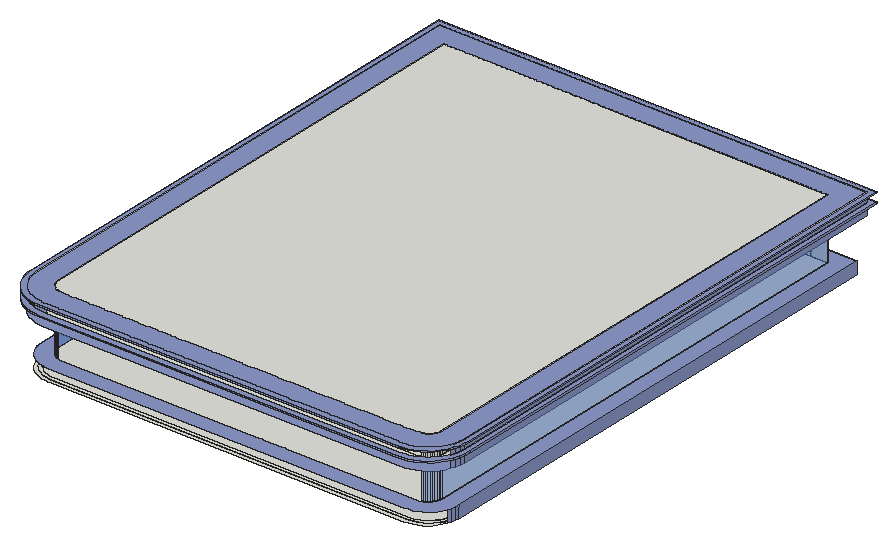
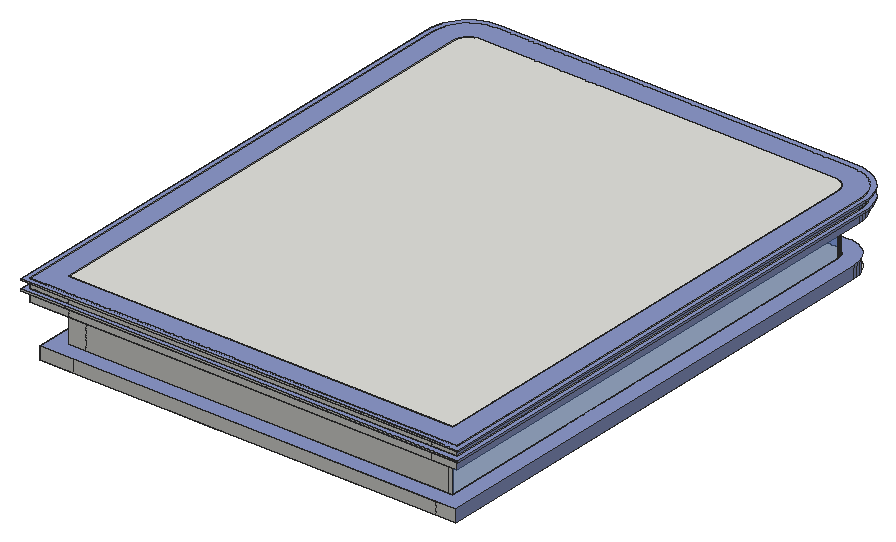
# SketchUp Ruby script. Lengths in inches.
U = 1.inch
M = Sketchup.active_model
def pt(a) = Geom::Point3d.new(a.map { |v| v * U })
def face(e, loops, mat)
  f = e.add_face(loops[0].map { |a| pt(a) })
  loops[1..].each { |l| e.add_face(l.map { |a| pt(a) }).erase! }
  f.material = f.back_material = mat if mat
  f
end
# faces: each face lists its corners as indices into pts; further lists are holes
def faces(e, pts, list, mat = nil) = list.each { |f| face(e, (f[0].is_a?(Array) ? f : [f]).map { |l| l.map { |i| pts[i] } }, mat) }
# xy, xz, yz: faces in a plane at the given z, y or x. An outline is a flat list of corners, or four numbers for a rectangle; further outlines are holes
def ring(l) = l.size == 4 ? [[l[0], l[1]], [l[2], l[1]], [l[2], l[3]], [l[0], l[3]]] : l.each_slice(2).to_a
def flat(e, list, mat, &to3) = list.each { |f| face(e, (f[0].is_a?(Array) ? f : [f]).map { |l| ring(l).map { |u, v| to3.(u, v) } }, mat) }
def xy(e, z, list, mat = nil) = flat(e, list, mat) { |x, y| [x, y, z] }
def xz(e, y, list, mat = nil) = flat(e, list, mat) { |x, z| [x, y, z] }
def yz(e, x, list, mat = nil) = flat(e, list, mat) { |y, z| [x, y, z] }
def lines(e, pts, list) = list.each { |a, b| e.add_line(pt(pts[a]), pt(pts[b])) }
# prism: a flat outline (further loops are holes) pulled along v
def prism(e, loops, v, mat = nil)
  f = face(e, loops, mat); d = Geom::Vector3d.new(v.map { |x| x * U })
  f.pushpull(f.normal.samedirection?(d) ? d.length : -d.length)
end
def box(e, o, s, mat = nil) = prism(e, [[o, [o[0] + s[0], o[1], o[2]], [o[0] + s[0], o[1] + s[1], o[2]], [o[0], o[1] + s[1], o[2]]]], [0, 0, s[2]], mat)
def at(x, y, z, deg = 0) = Geom::Transformation.translation(pt([x, y, z])) * Geom::Transformation.rotation(ORIGIN, Z_AXIS, deg.degrees)
def axes(o, x, y, z) = Geom::Transformation.new([*x, 0, *y, 0, *z, 0, *pt(o).to_a, 1])
def part(name) = M.definitions.add(name)
# library, detail: a bought-in or finely detailed component or shape, given as its bounding box
def library(name, o, s) = part(name).tap { |d| box(d.entities, o, s) }
def detail(e, o, s) = box(e.add_group.entities, o, s)
def put(e, d, t, mat = nil) = e.add_instance(d, t).tap { |i| i.material = mat if mat }
def group(e, t, mat = nil) = e.add_group.tap { |g| g.transformation = t; g.material = mat if mat }.entities
root = M.entities
M.materials.add("0326 AP 7207 CLASSIC PURPLE").color = [140, 152, 201]
M.materials.add("[Translucent Glass Blue]").color = [100, 149, 237]
M.materials["[Translucent Glass Blue]"].alpha = 0.5
xy(root,372,[[[167.6875,42.4375,166.41,42.52,163.74,42.7,159.87,43.47,157.41,44.3,156.125,44.74,152.58,46.49,149.29,48.68,146.32,51.29,143.71,54.26,141.52,57.55,139.77,61.09,138.5,64.84,137.73,68.71,137.47,72.66,137.47,233.75,247.2,233.75,247.2,141.25,257.02,141.25,257.02,224.35,364.41,224.35,364.41,86.25,517.41,86.25,517.41,566.25,550.66,566.25,550.66,72.66,550.4,68.71,549.63,64.84,548.36,61.09,546.61,57.55,544.41,54.26,541.81,51.29,538.83,48.68,535.55,46.49,532,44.74,528.26,43.47,524.38,42.7,520.4375,42.4375],[167.8,45.71,520.4375,45.71,523.96,45.9375,527.41,46.625,530.75,47.76,533.91,49.32,536.84,51.28,539.49,53.6,541.82,56.25,543.78,59.18,545.34,62.34,546.47,65.68,547.16,69.14,547.39,72.66,547.39,176.17,544.33,176.17,544.33,72.66,544.12,69.54,543.51,66.47,542.51,63.51,541.125,60.71,539.39,58.11,537.33,55.76,534.98,53.7,532.38,51.97,529.58,50.59,526.62,49.58,523.56,48.97,520.4375,48.77,167.9,48.77,166.82,48.84,164.57,48.98,161.51,49.59,159.44,50.3,158.55,50.6,155.75,51.98,153.15,53.71,150.81,55.77,148.75,58.12,147.01,60.72,145.63,63.52,144.625,66.48,144.02,69.54,143.8,72.86,143.8,227.42,140.74,230.48,140.74,72.76,140.98,69.14,141.66,65.68,142.8,62.35,144.36,59.1875,146.3125,56.26,148.64,53.61,151.29,51.28,154.22,49.32,157.38,47.77,158.46,47.4,160.72,46.63,164.17,45.95,166.62,45.78]],[364.41,86.25,373.41,566.25],[373.41,86.25,508.41,95.25],[508.41,86.25,517.41,95.25],[373.41,95.25,508.41,557.25],
  [508.41,95.25,517.41,566.25],[247.2,141.25,257.02,566.25],[257.02,224.35,364.41,238.8],[137.47,233.75,157.41,566.25],[157.41,233.75,166.41,566.25],
  [166.41,233.75,247.2,252.68],[257.02,238.8,364.41,566.25],[166.41,252.68,247.2,566.25],[373.41,557.25,508.41,566.25]])
xy(root,372.8125,[[167.8,45.71,166.62,45.78,164.17,45.95,160.72,46.63,158.46,47.4,157.38,47.77,154.22,49.32,151.29,51.28,148.64,53.61,146.3125,56.26,144.36,59.1875,142.8,62.35,141.66,65.68,140.98,69.14,140.74,72.76,140.74,230.48,143.8,227.42,143.8,72.86,144.02,69.54,144.625,66.48,145.63,63.52,147.01,60.72,148.75,58.12,150.81,55.77,153.15,53.71,155.75,51.98,158.55,50.6,159.44,50.3,161.51,49.59,164.57,48.98,166.82,48.84,167.9,48.77,520.4375,48.77,523.56,48.97,526.62,49.58,529.58,50.59,532.38,51.97,534.98,53.7,537.33,55.76,539.39,58.11,541.125,60.71,542.51,63.51,543.51,66.47,544.12,69.54,544.33,72.66,544.33,176.17,547.39,176.17,547.39,72.66,547.16,69.14,546.47,65.68,545.34,62.34,543.78,59.18,541.82,56.25,539.49,53.6,536.84,51.28,533.91,49.32,530.75,47.76,527.41,46.625,523.96,45.9375,520.4375,45.71]])
xy(root,384,[[168.22,58.64,165.86,58.8,164.07,59.15,162.62,59.65,162.34,59.74,160.7,60.55,159.18,61.57,157.8,62.77,156.6,64.15,155.58,65.67,154.77,67.31,154.1875,69.04,153.83,70.83,153.68,73.1875,153.68,550.04,534.45,550.04,534.45,72.66,534.33,70.83,533.97,69.03,533.38,67.29,532.57,65.65,531.56,64.125,530.35,62.75,528.97,61.54,527.44,60.52,525.8,59.71,524.06,59.12,522.27,58.76,520.4375,58.64]])
xy(root,384,[[[167.6875,42.4375,520.4375,42.4375,524.38,42.7,528.26,43.47,532,44.74,535.55,46.49,538.83,48.68,541.81,51.29,544.41,54.26,546.61,57.55,548.36,61.09,549.63,64.84,550.4,68.71,550.66,72.66,550.66,566.25,137.47,566.25,137.47,72.66,137.73,68.71,138.5,64.84,139.77,61.09,141.52,57.55,143.71,54.26,146.32,51.29,149.29,48.68,152.58,46.49,156.125,44.74,157.41,44.3,159.87,43.47,163.74,42.7],[168.22,58.64,165.86,58.8,164.07,59.15,162.62,59.65,162.34,59.74,160.7,60.55,159.18,61.57,157.8,62.77,156.6,64.15,155.58,65.67,154.77,67.31,154.1875,69.04,153.83,70.83,153.68,73.1875,153.68,550.04,534.45,550.04,534.45,72.66,534.33,70.83,533.97,69.03,533.38,67.29,532.57,65.65,531.56,64.125,530.35,62.75,528.97,61.54,527.44,60.52,525.8,59.71,524.06,59.12,522.27,58.76,520.4375,58.64]]],"0326 AP 7207 CLASSIC PURPLE")
xy(root,420.75,[[[168.01,52.13,165.01,52.33,162.38,52.85,160.52,53.48,159.84,53.72,157.4375,54.9,155.21,56.39,153.19,58.16,151.42,60.18,149.93,62.41,148.75,64.8125,147.89,67.35,147.36,69.98,147.17,72.97,147.17,556.55,540.96,556.55,540.96,72.66,540.78,69.98,540.26,67.34,539.4,64.8,538.21,62.4,536.72,60.16,534.95,58.15,532.93,56.375,530.7,54.88,528.29,53.7,525.75,52.83,523.12,52.31,520.4375,52.13],[168.22,58.64,520.4375,58.64,522.27,58.76,524.06,59.12,525.8,59.71,527.44,60.52,528.97,61.54,530.35,62.75,531.56,64.125,532.57,65.65,533.38,67.29,533.97,69.03,534.33,70.83,534.45,72.66,534.45,550.04,153.68,550.04,153.68,73.1875,153.83,70.83,154.1875,69.04,154.77,67.31,155.58,65.67,156.6,64.15,157.8,62.77,159.18,61.57,160.7,60.55,162.34,59.74,162.62,59.65,164.07,59.15,165.86,58.8]]],"0326 AP 7207 CLASSIC PURPLE")
xy(root,423.4375,[[[168.01,52.13,520.4375,52.13,523.12,52.31,525.75,52.83,528.29,53.7,530.7,54.88,532.93,56.375,534.95,58.15,536.72,60.16,538.21,62.4,539.4,64.8,540.26,67.34,540.78,69.98,540.96,72.66,540.96,556.55,147.17,556.55,147.17,72.97,147.36,69.98,147.89,67.35,148.75,64.8125,149.93,62.41,151.42,60.18,153.19,58.16,155.21,56.39,157.4375,54.9,159.84,53.72,160.52,53.48,162.38,52.85,165.01,52.33],[168.22,58.64,165.86,58.8,164.07,59.15,162.62,59.65,162.34,59.74,160.7,60.55,159.18,61.57,157.8,62.77,156.6,64.15,155.58,65.67,154.77,67.31,154.1875,69.04,153.83,70.83,153.68,73.1875,153.68,550.04,534.45,550.04,534.45,72.66,534.33,70.83,533.97,69.03,533.38,67.29,532.57,65.65,531.56,64.125,530.35,62.75,528.97,61.54,527.44,60.52,525.8,59.71,524.06,59.12,522.27,58.76,520.4375,58.64]]])
xy(root,423.4375,[[[167.51,37.02,163.03,37.3125,158.46,38.22,155.67,39.17,154.05,39.72,149.86,41.78,145.99,44.375,142.48,47.45,139.41,50.95,136.82,54.83,134.75,59.01,133.25,63.43,132.34,68,132.05,72.48,132.05,571.67,556.08,571.67,556.08,72.66,555.77,68,554.86,63.43,553.36,59.02,551.3,54.84,548.71,50.96,545.64,47.46,542.13,44.38,538.26,41.79,534.08,39.73,529.66,38.23,525.09,37.32,520.4375,37.02],[168.01,52.13,520.4375,52.13,523.12,52.31,525.75,52.83,528.29,53.7,530.7,54.88,532.93,56.375,534.95,58.15,536.72,60.16,538.21,62.4,539.4,64.8,540.26,67.34,540.78,69.98,540.96,72.66,540.96,556.55,147.17,556.55,147.17,72.97,147.36,69.98,147.89,67.35,148.75,64.8125,149.93,62.41,151.42,60.18,153.19,58.16,155.21,56.39,157.4375,54.9,159.84,53.72,160.52,53.48,162.38,52.85,165.01,52.33]]],"0326 AP 7207 CLASSIC PURPLE")
xy(root,433.9375,[[[167.34,31.9,162.36,32.22,157.13,33.26,154.02,34.32,152.08,34.98,147.3,37.34,142.86,40.3,138.85,43.82,135.33,47.83,132.37,52.26,130.01,57.05,128.29,62.1,127.25,67.33,126.93,72.3125,126.93,576.79,561.2,576.79,561.2,72.66,560.85,67.34,559.81,62.11,558.1,57.06,555.74,52.28,552.78,47.84,549.26,43.83,545.25,40.32,540.82,37.36,536.04,35,530.99,33.28,525.76,32.24,520.4375,31.9],[167.51,37.02,520.4375,37.02,525.09,37.32,529.66,38.23,534.08,39.73,538.26,41.79,542.13,44.38,545.64,47.46,548.71,50.96,551.3,54.84,553.36,59.02,554.86,63.43,555.77,68,556.08,72.66,556.08,571.67,132.05,571.67,132.05,72.48,132.34,68,133.25,63.43,134.75,59.01,136.82,54.83,139.41,50.95,142.48,47.45,145.99,44.375,149.86,41.78,154.05,39.72,155.67,39.17,158.46,38.22,163.03,37.3125]]],"0326 AP 7207 CLASSIC PURPLE")
xy(root,435.625,[[[167.34,31.9,520.4375,31.9,525.76,32.24,530.99,33.28,536.04,35,540.82,37.36,545.25,40.32,549.26,43.83,552.78,47.84,555.74,52.28,558.1,57.06,559.81,62.11,560.85,67.34,561.2,72.66,561.2,576.79,126.93,576.79,126.93,72.3125,127.25,67.33,128.29,62.1,130.01,57.05,132.37,52.26,135.33,47.83,138.85,43.82,142.86,40.3,147.3,37.34,152.08,34.98,154.02,34.32,157.13,33.26,162.36,32.22],[167.51,37.02,163.03,37.3125,158.46,38.22,155.67,39.17,154.05,39.72,149.86,41.78,145.99,44.375,142.48,47.45,139.41,50.95,136.82,54.83,134.75,59.01,133.25,63.43,132.34,68,132.05,72.48,132.05,571.67,556.08,571.67,556.08,72.66,555.77,68,554.86,63.43,553.36,59.02,551.3,54.84,548.71,50.96,545.64,47.46,542.13,44.38,538.26,41.79,534.08,39.73,529.66,38.23,525.09,37.32,520.4375,37.02]]],"0326 AP 7207 CLASSIC PURPLE")
xy(root,443.3125,[[[167.34,31.9,162.36,32.22,157.13,33.26,154.02,34.32,152.08,34.98,147.3,37.34,142.86,40.3,138.85,43.82,135.33,47.83,132.37,52.26,130.01,57.05,128.29,62.1,127.25,67.33,126.93,72.3125,126.93,576.79,561.2,576.79,561.2,72.66,560.85,67.34,559.81,62.11,558.1,57.06,555.74,52.28,552.78,47.84,549.26,43.83,545.25,40.32,540.82,37.36,536.04,35,530.99,33.28,525.76,32.24,520.4375,31.9],[167.51,37.02,520.4375,37.02,525.09,37.32,529.66,38.23,534.08,39.73,538.26,41.79,542.13,44.38,545.64,47.46,548.71,50.96,551.3,54.84,553.36,59.02,554.86,63.43,555.77,68,556.08,72.66,556.08,571.67,132.05,571.67,132.05,72.48,132.34,68,133.25,63.43,134.75,59.01,136.82,54.83,139.41,50.95,142.48,47.45,145.99,44.375,149.86,41.78,154.05,39.72,155.67,39.17,158.46,38.22,163.03,37.3125]]],"0326 AP 7207 CLASSIC PURPLE")
xy(root,444.625,[[168.22,58.64,520.4375,58.64,522.27,58.76,524.06,59.12,525.8,59.71,527.44,60.52,528.97,61.54,530.35,62.75,531.56,64.125,532.57,65.65,533.38,67.29,533.97,69.03,534.33,70.83,534.45,72.66,534.45,550.04,153.68,550.04,153.68,73.1875,153.83,70.83,154.1875,69.04,154.77,67.31,155.58,65.67,156.6,64.15,157.8,62.77,159.18,61.57,160.7,60.55,162.34,59.74,162.62,59.65,164.07,59.15,165.86,58.8]])
xy(root,444.625,[[[167.34,31.9,520.4375,31.9,525.76,32.24,530.99,33.28,536.04,35,540.82,37.36,545.25,40.32,549.26,43.83,552.78,47.84,555.74,52.28,558.1,57.06,559.81,62.11,560.85,67.34,561.2,72.66,561.2,576.79,126.93,576.79,126.93,72.3125,127.25,67.33,128.29,62.1,130.01,57.05,132.37,52.26,135.33,47.83,138.85,43.82,142.86,40.3,147.3,37.34,152.08,34.98,154.02,34.32,157.13,33.26,162.36,32.22],[167.51,37.02,163.03,37.3125,158.46,38.22,155.67,39.17,154.05,39.72,149.86,41.78,145.99,44.375,142.48,47.45,139.41,50.95,136.82,54.83,134.75,59.01,133.25,63.43,132.34,68,132.05,72.48,132.05,571.67,556.08,571.67,556.08,72.66,555.77,68,554.86,63.43,553.36,59.02,551.3,54.84,548.71,50.96,545.64,47.46,542.13,44.38,538.26,41.79,534.08,39.73,529.66,38.23,525.09,37.32,520.4375,37.02]],[[167.51,37.02,520.4375,37.02,525.09,37.32,529.66,38.23,534.08,39.73,538.26,41.79,542.13,44.38,545.64,47.46,548.71,50.96,551.3,54.84,553.36,59.02,554.86,63.43,555.77,68,556.08,72.66,556.08,571.67,132.05,571.67,132.05,72.48,132.34,68,133.25,63.43,134.75,59.01,136.82,54.83,139.41,50.95,142.48,47.45,145.99,44.375,149.86,41.78,154.05,39.72,155.67,39.17,158.46,38.22,163.03,37.3125],[168.22,58.64,165.86,58.8,164.07,59.15,162.62,59.65,162.34,59.74,160.7,60.55,159.18,61.57,157.8,62.77,156.6,64.15,155.58,65.67,154.77,67.31,154.1875,69.04,153.83,70.83,153.68,73.1875,153.68,550.04,534.45,550.04,534.45,72.66,534.33,70.83,533.97,69.03,533.38,67.29,532.57,65.65,531.56,64.125,530.35,62.75,528.97,61.54,527.44,60.52,525.8,59.71,524.06,59.12,522.27,58.76,520.4375,58.64]]],"0326 AP 7207 CLASSIC PURPLE")
xz(root,176.17,[[544.33,372,547.39,372.8125]])
xz(root,550.04,[[153.68,384,157.41,420.75],[157.41,384,517.41,420.75],[517.41,384,534.45,420.75],[153.68,420.75,157.41,423.4375],[157.41,420.75,517.41,423.4375],
  [517.41,420.75,534.45,423.4375],[153.68,423.4375,157.41,444.625],[157.41,423.4375,517.41,444.625],[517.41,423.4375,534.45,444.625]])
xz(root,556.55,[[147.17,420.75,157.41,423.4375],[157.41,420.75,517.41,423.4375],[517.41,420.75,540.96,423.4375]])
xz(root,566.25,[[137.47,372,157.41,384],[157.41,372,517.41,384],[517.41,372,550.66,384]])
xz(root,571.67,[[132.05,423.4375,157.41,433.9375],[157.41,423.4375,517.41,433.9375],[517.41,423.4375,556.08,433.9375],[132.05,433.9375,157.41,435.625],[157.41,433.9375,517.41,435.625],
  [517.41,433.9375,556.08,435.625],[132.05,435.625,157.41,443.3125],[157.41,435.625,517.41,443.3125],[517.41,435.625,556.08,443.3125],[132.05,443.3125,157.41,444.625],
  [157.41,443.3125,517.41,444.625],[517.41,443.3125,556.08,444.625]])
xz(root,576.79,[[126.93,433.9375,157.41,435.625],[157.41,433.9375,517.41,435.625],[517.41,433.9375,561.2,435.625],[126.93,443.3125,157.41,444.625],[157.41,443.3125,517.41,444.625],
  [517.41,443.3125,561.2,444.625]])
yz(root,126.93,[[72.3125,433.9375,576.79,435.625],[72.3125,443.3125,576.79,444.625]],"0326 AP 7207 CLASSIC PURPLE")
yz(root,132.05,[[72.48,433.9375,571.67,435.625],[72.48,443.3125,571.67,444.625]])
yz(root,132.05,[[72.48,423.4375,571.67,433.9375],[72.48,435.625,571.67,443.3125]],"0326 AP 7207 CLASSIC PURPLE")
yz(root,137.47,[[72.66,372,566.25,384]],"0326 AP 7207 CLASSIC PURPLE")
yz(root,140.74,[[72.76,372,230.48,372.8125]])
yz(root,143.8,[[72.86,372,227.42,372.8125]])
yz(root,147.17,[[72.97,420.75,556.55,423.4375]],"0326 AP 7207 CLASSIC PURPLE")
yz(root,153.68,[[73.1875,420.75,550.04,423.4375],[73.1875,423.4375,550.04,444.625]])
yz(root,153.68,[[73.1875,384,550.04,420.75]],"[Translucent Glass Blue]")
yz(root,534.45,[[72.66,420.75,550.04,423.4375],[72.66,423.4375,550.04,444.625]])
yz(root,534.45,[[72.66,384,550.04,420.75]],"[Translucent Glass Blue]")
yz(root,540.96,[[72.66,420.75,556.55,423.4375]],"0326 AP 7207 CLASSIC PURPLE")
yz(root,544.33,[[72.66,372,176.17,372.8125]])
yz(root,547.39,[[72.66,372,176.17,372.8125]])
yz(root,550.66,[[72.66,372,566.25,384]],"0326 AP 7207 CLASSIC PURPLE")
yz(root,556.08,[[72.66,433.9375,571.67,435.625],[72.66,443.3125,571.67,444.625]])
yz(root,556.08,[[72.66,423.4375,571.67,433.9375],[72.66,435.625,571.67,443.3125]],"0326 AP 7207 CLASSIC PURPLE")
yz(root,561.2,[[72.66,433.9375,576.79,435.625],[72.66,443.3125,576.79,444.625]],"0326 AP 7207 CLASSIC PURPLE")
p = [[147.01,60.72,372],[148.75,58.12,372],[148.75,58.12,372.8125],[147.01,60.72,372.8125],[539.39,58.11,372],[541.125,60.71,372],
  [541.125,60.71,372.8125],[539.39,58.11,372.8125],[144.36,59.1875,372],[142.8,62.35,372],[142.8,62.35,372.8125],[144.36,59.1875,372.8125],
  [545.34,62.34,372],[543.78,59.18,372],[543.78,59.18,372.8125],[545.34,62.34,372.8125],[145.63,63.52,372],[145.63,63.52,372.8125],
  [542.51,63.51,372],[542.51,63.51,372.8125],[139.77,61.09,384],[138.5,64.84,384],[138.5,64.84,372],[139.77,61.09,372],
  [549.63,64.84,384],[548.36,61.09,384],[548.36,61.09,372],[549.63,64.84,372],[141.66,65.68,372],[141.66,65.68,372.8125],
  [546.47,65.68,372],[546.47,65.68,372.8125],[144.625,66.48,372],[144.625,66.48,372.8125],[543.51,66.47,372],[543.51,66.47,372.8125],
  [137.73,68.71,384],[137.73,68.71,372],[550.4,68.71,384],[550.4,68.71,372],[140.98,69.14,372],[140.98,69.14,372.8125],
  [547.16,69.14,372],[547.16,69.14,372.8125],[144.02,69.54,372],[144.02,69.54,372.8125],[544.12,69.54,372],[544.12,69.54,372.8125],
  [137.47,72.66,384],[137.47,72.66,372],[550.66,72.66,384],[550.66,72.66,372],[140.74,72.76,372],[140.74,72.76,372.8125],
  [547.39,72.66,372],[547.39,72.66,372.8125],[143.8,72.86,372],[143.8,72.86,372.8125],[544.33,72.66,372],[544.33,72.66,372.8125],
  [140.74,230.48,372],[143.8,227.42,372],[143.8,227.42,372.8125],[140.74,230.48,372.8125],[524.06,59.12,384],[525.8,59.71,384],
  [525.8,59.71,420.75],[524.06,59.12,420.75],[162.62,59.65,384],[164.07,59.15,384],[164.07,59.15,420.75],[162.62,59.65,420.75],
  [162.34,59.74,384],[162.34,59.74,420.75],[160.7,60.55,384],[160.7,60.55,420.75],[527.44,60.52,384],[527.44,60.52,420.75],
  [528.97,61.54,384],[528.97,61.54,420.75],[159.18,61.57,384],[159.18,61.57,420.75],[530.35,62.75,384],[530.35,62.75,420.75],
  [157.8,62.77,384],[157.8,62.77,420.75],[531.56,64.125,384],[531.56,64.125,420.75],[156.6,64.15,384],[156.6,64.15,420.75],
  [155.58,65.67,384],[155.58,65.67,420.75],[532.57,65.65,384],[532.57,65.65,420.75],[533.38,67.29,384],[533.38,67.29,420.75],
  [154.77,67.31,384],[154.77,67.31,420.75],[154.1875,69.04,384],[154.1875,69.04,420.75],[533.97,69.03,384],[533.97,69.03,420.75],
  [153.83,70.83,384],[153.83,70.83,420.75],[534.33,70.83,384],[534.33,70.83,420.75],[153.68,73.1875,384],[153.68,73.1875,420.75],
  [534.45,72.66,384],[534.45,72.66,420.75],[525.8,59.71,423.4375],[524.06,59.12,423.4375],[164.07,59.15,423.4375],[162.62,59.65,423.4375],
  [162.34,59.74,423.4375],[160.7,60.55,423.4375],[527.44,60.52,423.4375],[151.42,60.18,423.4375],[149.93,62.41,423.4375],[149.93,62.41,420.75],
  [151.42,60.18,420.75],[538.21,62.4,423.4375],[536.72,60.16,423.4375],[536.72,60.16,420.75],[538.21,62.4,420.75],[528.97,61.54,423.4375],
  [159.18,61.57,423.4375],[530.35,62.75,423.4375],[157.8,62.77,423.4375],[148.75,64.8125,423.4375],[148.75,64.8125,420.75],[539.4,64.8,423.4375],
  [539.4,64.8,420.75],[531.56,64.125,423.4375],[156.6,64.15,423.4375],[155.58,65.67,423.4375],[532.57,65.65,423.4375],[147.89,67.35,423.4375],
  [147.89,67.35,420.75],[540.26,67.34,423.4375],[540.26,67.34,420.75],[533.38,67.29,423.4375],[154.77,67.31,423.4375],[154.1875,69.04,423.4375],
  [533.97,69.03,423.4375],[540.78,69.98,423.4375],[540.78,69.98,420.75],[147.36,69.98,423.4375],[147.36,69.98,420.75],[153.83,70.83,423.4375],
  [534.33,70.83,423.4375],[147.17,72.97,423.4375],[147.17,72.97,420.75],[540.96,72.66,423.4375],[540.96,72.66,420.75],[153.68,73.1875,423.4375],
  [534.45,72.66,423.4375],[133.25,63.43,423.4375],[134.75,59.01,423.4375],[134.75,59.01,433.9375],[133.25,63.43,433.9375],[553.36,59.02,423.4375],
  [554.86,63.43,423.4375],[554.86,63.43,433.9375],[553.36,59.02,433.9375],[524.06,59.12,444.625],[525.8,59.71,444.625],[162.62,59.65,444.625],
  [164.07,59.15,444.625],[162.34,59.74,444.625],[160.7,60.55,444.625],[527.44,60.52,444.625],[528.97,61.54,444.625],[159.18,61.57,444.625],
  [530.35,62.75,444.625],[157.8,62.77,444.625],[531.56,64.125,444.625],[156.6,64.15,444.625],[132.34,68,423.4375],[132.34,68,433.9375],
  [555.77,68,423.4375],[555.77,68,433.9375],[155.58,65.67,444.625],[532.57,65.65,444.625],[533.38,67.29,444.625],[154.77,67.31,444.625],
  [154.1875,69.04,444.625],[533.97,69.03,444.625],[132.05,72.48,423.4375],[132.05,72.48,433.9375],[556.08,72.66,423.4375],[556.08,72.66,433.9375],
  [153.83,70.83,444.625],[534.33,70.83,444.625],[153.68,73.1875,444.625],[534.45,72.66,444.625],[128.29,62.1,433.9375],[130.01,57.05,433.9375],
  [130.01,57.05,435.625],[128.29,62.1,435.625],[558.1,57.06,433.9375],[559.81,62.11,433.9375],[559.81,62.11,435.625],[558.1,57.06,435.625],
  [133.25,63.43,435.625],[134.75,59.01,435.625],[553.36,59.02,435.625],[554.86,63.43,435.625],[127.25,67.33,433.9375],[127.25,67.33,435.625],
  [560.85,67.34,433.9375],[560.85,67.34,435.625],[132.34,68,435.625],[555.77,68,435.625],[126.93,72.3125,433.9375],[126.93,72.3125,435.625],
  [561.2,72.66,433.9375],[561.2,72.66,435.625],[132.05,72.48,435.625],[556.08,72.66,435.625],[134.75,59.01,443.3125],[133.25,63.43,443.3125],
  [554.86,63.43,443.3125],[553.36,59.02,443.3125],[132.34,68,443.3125],[555.77,68,443.3125],[132.05,72.48,443.3125],[556.08,72.66,443.3125],
  [128.29,62.1,443.3125],[130.01,57.05,443.3125],[130.01,57.05,444.625],[128.29,62.1,444.625],[558.1,57.06,443.3125],[559.81,62.11,443.3125],
  [559.81,62.11,444.625],[558.1,57.06,444.625],[133.25,63.43,444.625],[134.75,59.01,444.625],[553.36,59.02,444.625],[554.86,63.43,444.625],
  [127.25,67.33,443.3125],[127.25,67.33,444.625],[560.85,67.34,443.3125],[560.85,67.34,444.625],[132.34,68,444.625],[555.77,68,444.625],
  [126.93,72.3125,443.3125],[126.93,72.3125,444.625],[561.2,72.66,443.3125],[561.2,72.66,444.625],[132.05,72.48,444.625],[556.08,72.66,444.625],
  [172.74,559.92,372],[240.875,559.92,372],[263.35,559.92,372],[358.08,559.92,372],[523.74,559.92,372],[544.33,559.92,372],
  [169.68,562.98,372],[243.93,562.98,372],[260.29,562.98,372],[361.14,562.98,372],[520.68,562.98,372],[547.39,562.98,372]]
faces(root,p,[[0,1,2,3],[4,5,6,7],[8,9,10,11],[12,13,14,15],[16,0,3,17],[5,18,19,6],[9,28,29,10],[30,12,15,31],
  [32,16,17,33],[18,34,35,19],[28,40,41,29],[42,30,31,43],[44,32,33,45],[34,46,47,35],[40,52,53,41],[54,42,43,55],
  [56,44,45,57],[46,58,59,47],[60,61,62,63],[110,111,67,66],[112,113,71,70],[113,114,73,71],[114,115,75,73],[116,110,66,77],
  [125,116,77,79],[115,126,81,75],[127,125,79,83],[126,128,85,81],[133,127,83,87],[128,134,89,85],[134,135,91,89],[136,133,87,93],
  [141,136,93,95],[135,142,97,91],[142,143,99,97],[144,141,95,101],[143,149,103,99],[150,144,101,105],[149,155,107,103],[156,150,105,109],
  [110,111,165,166],[112,113,167,168],[113,114,169,167],[114,115,170,169],[116,110,166,171],[125,116,171,172],[115,126,173,170],[127,125,172,174],
  [126,128,175,173],[133,127,174,176],[128,134,177,175],[134,135,182,177],[136,133,176,183],[141,136,183,184],[135,142,185,182],[142,143,186,185],
  [144,141,184,187],[143,149,192,186],[150,144,187,193],[149,155,194,192],[156,150,193,195],[159,160,204,205],[163,164,206,207],[160,179,212,204],
  [181,163,207,213],[179,189,218,212],[191,181,213,219],[220,221,236,237],[222,223,238,239],[221,224,244,236],[225,222,239,245],[224,226,250,244],
  [227,225,245,251]])
faces(root,p,[[20,21,22,23],[24,25,26,27],[21,36,37,22],[38,24,27,39],[36,48,49,37],[50,38,39,51],[117,118,119,120],[121,122,123,124],
  [118,129,130,119],[131,121,124,132],[129,137,138,130],[139,131,132,140],[145,139,140,146],[137,147,148,138],[147,151,152,148],[153,145,146,154],
  [157,158,159,160],[161,162,163,164],[178,157,160,179],[162,180,181,163],[188,178,179,189],[180,190,191,181],[196,197,198,199],[200,201,202,203],
  [208,196,199,209],[201,210,211,202],[214,208,209,215],[210,216,217,211],[204,205,220,221],[206,207,222,223],[212,204,221,224],[207,213,225,222],
  [218,212,224,226],[213,219,227,225],[228,229,230,231],[232,233,234,235],[240,228,231,241],[233,242,243,234],[246,240,241,247],[242,248,249,243]],"0326 AP 7207 CLASSIC PURPLE")
faces(root,p,[[64,65,66,67],[68,69,70,71],[72,68,71,73],[74,72,73,75],[65,76,77,66],[76,78,79,77],[80,74,75,81],[78,82,83,79],
  [84,80,81,85],[82,86,87,83],[88,84,85,89],[90,88,89,91],[86,92,93,87],[92,94,95,93],[96,90,91,97],[98,96,97,99],
  [94,100,101,95],[102,98,99,103],[100,104,105,101],[106,102,103,107],[104,108,109,105]],"[Translucent Glass Blue]")
lines(root,p,[[252,253],[254,255],[256,257],[258,259],[260,261],[262,263]])
